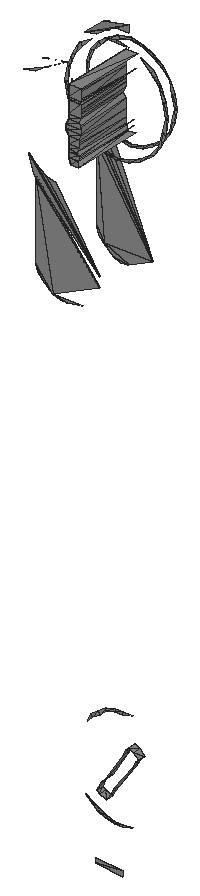
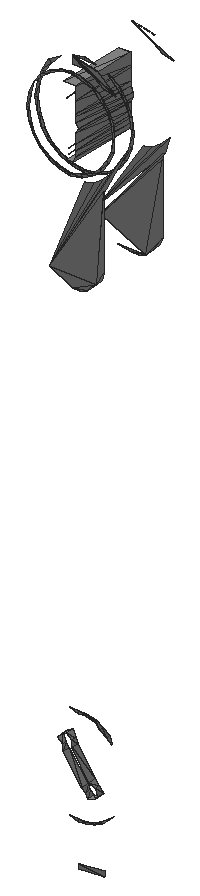
# SketchUp Ruby script. Lengths in inches.
U = 1.inch
M = Sketchup.active_model
def pt(a) = Geom::Point3d.new(a.map { |v| v * U })
def face(e, loops, mat)
  f = e.add_face(loops[0].map { |a| pt(a) })
  loops[1..].each { |l| e.add_face(l.map { |a| pt(a) }).erase! }
  f.material = f.back_material = mat if mat
  f
end
# faces: each face lists its corners as indices into pts; further lists are holes
def faces(e, pts, list, mat = nil) = list.each { |f| face(e, (f[0].is_a?(Array) ? f : [f]).map { |l| l.map { |i| pts[i] } }, mat) }
# xy, xz, yz: faces in a plane at the given z, y or x. An outline is a flat list of corners, or four numbers for a rectangle; further outlines are holes
def ring(l) = l.size == 4 ? [[l[0], l[1]], [l[2], l[1]], [l[2], l[3]], [l[0], l[3]]] : l.each_slice(2).to_a
def flat(e, list, mat, &to3) = list.each { |f| face(e, (f[0].is_a?(Array) ? f : [f]).map { |l| ring(l).map { |u, v| to3.(u, v) } }, mat) }
def xy(e, z, list, mat = nil) = flat(e, list, mat) { |x, y| [x, y, z] }
def xz(e, y, list, mat = nil) = flat(e, list, mat) { |x, z| [x, y, z] }
def yz(e, x, list, mat = nil) = flat(e, list, mat) { |y, z| [x, y, z] }
def lines(e, pts, list) = list.each { |a, b| e.add_line(pt(pts[a]), pt(pts[b])) }
# prism: a flat outline (further loops are holes) pulled along v
def prism(e, loops, v, mat = nil)
  f = face(e, loops, mat); d = Geom::Vector3d.new(v.map { |x| x * U })
  f.pushpull(f.normal.samedirection?(d) ? d.length : -d.length)
end
def box(e, o, s, mat = nil) = prism(e, [[o, [o[0] + s[0], o[1], o[2]], [o[0] + s[0], o[1] + s[1], o[2]], [o[0], o[1] + s[1], o[2]]]], [0, 0, s[2]], mat)
def at(x, y, z, deg = 0) = Geom::Transformation.translation(pt([x, y, z])) * Geom::Transformation.rotation(ORIGIN, Z_AXIS, deg.degrees)
def axes(o, x, y, z) = Geom::Transformation.new([*x, 0, *y, 0, *z, 0, *pt(o).to_a, 1])
def part(name) = M.definitions.add(name)
# library, detail: a bought-in or finely detailed component or shape, given as its bounding box
def library(name, o, s) = part(name).tap { |d| box(d.entities, o, s) }
def detail(e, o, s) = box(e.add_group.entities, o, s)
def put(e, d, t, mat = nil) = e.add_instance(d, t).tap { |i| i.material = mat if mat }
def group(e, t, mat = nil) = e.add_group.tap { |g| g.transformation = t; g.material = mat if mat }.entities
root = M.entities
M.materials.add("Material \#1").color = [140, 140, 140]
xy(root,161.124,[[359.541,200.864,359.541,201.153,359.571,200.864],[359.571,200.864,359.541,201.153,359.571,201.153]],"Material \#1")
xy(root,161.418,[[359.526,200.864,359.576,200.864,359.576,201.153],[359.526,200.864,359.576,201.153,359.526,201.153]],"Material \#1")
xz(root,200.833,[[359.551,160.635,359.494,160.65,359.609,160.65],[359.551,160.635,359.521,160.639,359.494,160.65],[359.494,160.65,359.42,161.042,359.679,160.743],[359.494,160.65,359.423,160.743,359.42,161.042],[359.494,160.65,359.449,160.688,359.423,160.743],
  [359.494,160.65,359.469,160.666,359.449,160.688],[359.449,160.688,359.433,160.714,359.423,160.743],[359.679,160.743,359.417,161.058,359.415,161.063],[359.679,160.743,359.419,161.053,359.417,161.058],[359.679,160.743,359.42,161.048,359.419,161.053],
  [359.423,160.743,359.42,160.775,359.42,161.042],[359.679,160.743,359.42,161.042,359.42,161.048],[359.682,160.775,359.39,161.133,359.422,161.099],[359.682,160.775,359.415,161.063,359.39,161.133],[359.682,160.775,359.422,161.099,359.46,161.073],
  [359.682,160.775,359.46,161.073,359.504,161.056],[359.368,161.427,359.46,161.469,359.422,161.443],[359.46,161.469,359.551,161.521,359.504,161.486],[359.448,161.495,359.497,161.514,359.551,161.521]],"Material \#1")
xz(root,200.864,[[359.541,161.124,359.561,161.146,359.531,161.146],[359.541,161.124,359.571,161.124,359.561,161.146],[359.531,161.146,359.567,161.153,359.526,161.153],[359.531,161.146,359.561,161.146,359.567,161.153],[359.526,161.153,359.567,161.153,359.567,161.17],
  [359.526,161.153,359.567,161.17,359.526,161.17],[359.526,161.17,359.561,161.177,359.531,161.177],[359.526,161.17,359.567,161.17,359.561,161.177],[359.531,161.177,359.561,161.177,359.571,161.205],[359.531,161.177,359.571,161.205,359.531,161.205],
  [359.531,161.205,359.571,161.205,359.571,161.231],[359.531,161.205,359.571,161.231,359.531,161.231],[359.531,161.231,359.579,161.251,359.524,161.251],[359.531,161.231,359.571,161.231,359.579,161.251],[359.524,161.251,359.579,161.251,359.579,161.272],
  [359.524,161.251,359.579,161.272,359.524,161.272],[359.524,161.272,359.571,161.293,359.531,161.293],[359.524,161.272,359.579,161.272,359.571,161.293],[359.531,161.293,359.576,161.308,359.526,161.308],[359.531,161.293,359.571,161.293,359.576,161.308],
  [359.526,161.308,359.576,161.308,359.576,161.356],[359.526,161.308,359.576,161.356,359.526,161.356],[359.526,161.356,359.57,161.359,359.533,161.359],[359.526,161.356,359.576,161.356,359.57,161.359],[359.533,161.359,359.57,161.359,359.57,161.367],
  [359.533,161.359,359.57,161.367,359.533,161.367],[359.533,161.367,359.576,161.37,359.526,161.37],[359.533,161.367,359.57,161.367,359.576,161.37],[359.526,161.37,359.576,161.37,359.576,161.418],[359.526,161.37,359.576,161.418,359.526,161.418]],"Material \#1")
xz(root,201.082,[[359.551,161.051,359.551,161.058,359.498,161.058],[359.551,161.051,359.603,161.065,359.551,161.058],[359.551,161.051,359.605,161.058,359.603,161.065],[359.498,161.058,359.499,161.065,359.448,161.08],[359.498,161.058,359.551,161.058,359.499,161.065],
  [359.605,161.058,359.651,161.087,359.603,161.065],[359.605,161.058,359.655,161.08,359.651,161.087],[359.499,161.065,359.451,161.087,359.448,161.08],[359.448,161.08,359.451,161.087,359.405,161.115],[359.655,161.08,359.693,161.12,359.651,161.087],
  [359.655,161.08,359.698,161.115,359.693,161.12],[359.451,161.087,359.41,161.12,359.405,161.115],[359.405,161.115,359.41,161.12,359.372,161.161],[359.698,161.115,359.725,161.165,359.693,161.12],[359.698,161.115,359.731,161.161,359.725,161.165],
  [359.41,161.12,359.378,161.165,359.372,161.161],[359.372,161.161,359.378,161.165,359.351,161.214],[359.731,161.161,359.745,161.216,359.725,161.165],[359.731,161.161,359.751,161.214,359.745,161.216],[359.378,161.165,359.358,161.216,359.351,161.214],
  [359.351,161.214,359.358,161.216,359.344,161.271],[359.751,161.214,359.751,161.271,359.745,161.216],[359.751,161.214,359.758,161.271,359.751,161.271],[359.358,161.216,359.351,161.271,359.344,161.271],[359.344,161.271,359.351,161.271,359.351,161.328],
  [359.351,161.271,359.358,161.326,359.351,161.328],[359.751,161.271,359.758,161.271,359.745,161.326],[359.758,161.271,359.751,161.328,359.745,161.326],[359.358,161.326,359.372,161.381,359.351,161.328],[359.358,161.326,359.378,161.378,359.372,161.381],
  [359.745,161.326,359.751,161.328,359.725,161.378],[359.751,161.328,359.731,161.381,359.725,161.378],[359.378,161.378,359.405,161.427,359.372,161.381],[359.378,161.378,359.41,161.422,359.405,161.427],[359.725,161.378,359.731,161.381,359.693,161.422],
  [359.731,161.381,359.698,161.427,359.693,161.422],[359.41,161.422,359.448,161.462,359.405,161.427],[359.41,161.422,359.451,161.456,359.448,161.462],[359.693,161.422,359.698,161.427,359.651,161.456],[359.698,161.427,359.655,161.462,359.651,161.456],
  [359.451,161.456,359.498,161.484,359.448,161.462],[359.451,161.456,359.499,161.477,359.498,161.484],[359.651,161.456,359.655,161.462,359.603,161.477],[359.655,161.462,359.605,161.484,359.603,161.477],[359.499,161.477,359.551,161.491,359.498,161.484],
  [359.499,161.477,359.551,161.484,359.551,161.491],[359.603,161.477,359.605,161.484,359.551,161.484],[359.551,161.484,359.605,161.484,359.551,161.491]],"Material \#1")
xz(root,201.113,[[359.551,158.424,359.551,158.435,359.443,158.434],[359.443,158.434,359.551,158.435,359.444,158.445],[359.551,158.596,359.551,158.607,359.515,158.599],[359.551,158.596,359.585,158.61,359.551,158.607],[359.515,158.599,359.517,158.61,359.481,158.609],
  [359.515,158.599,359.551,158.607,359.517,158.61],[359.481,158.609,359.485,158.62,359.45,158.625],[359.481,158.609,359.517,158.61,359.485,158.62],[359.485,158.62,359.455,158.635,359.45,158.625],[359.45,158.625,359.455,158.635,359.422,158.646],
  [359.455,158.635,359.429,158.655,359.422,158.646],[359.422,158.646,359.429,158.655,359.398,158.672],[359.406,158.94,359.429,158.964,359.422,158.973],[359.429,158.964,359.45,158.994,359.422,158.973],[359.429,158.964,359.455,158.984,359.45,158.994],
  [359.455,158.984,359.481,159.01,359.45,158.994],[359.455,158.984,359.485,158.999,359.481,159.01],[359.485,158.999,359.515,159.019,359.481,159.01],[359.485,158.999,359.517,159.009,359.515,159.019],[359.517,159.009,359.551,159.023,359.515,159.019],
  [359.517,159.009,359.551,159.012,359.551,159.023],[359.551,159.012,359.587,159.019,359.551,159.023]],"Material \#1")
xz(root,201.144,[[359.551,160.635,359.449,160.688,359.494,160.65],[359.551,160.635,359.654,160.688,359.449,160.688],[359.551,160.635,359.494,160.65,359.521,160.639],[359.494,160.65,359.449,160.688,359.469,160.666],[359.654,160.688,359.318,161.238,359.415,161.063],
  [359.654,160.688,359.39,161.133,359.318,161.238],[359.654,160.688,359.422,161.099,359.39,161.133],[359.654,160.688,359.415,161.063,359.417,161.058],[359.654,160.688,359.417,161.058,359.419,161.053],[359.654,160.688,359.419,161.053,359.42,161.048],
  [359.449,160.688,359.42,161.042,359.423,160.743],[359.449,160.688,359.42,161.048,359.42,161.042],[359.449,160.688,359.654,160.688,359.42,161.048],[359.654,160.688,359.46,161.073,359.422,161.099],[359.449,160.688,359.423,160.743,359.433,160.714],
  [359.654,160.688,359.504,161.056,359.46,161.073],[359.423,160.743,359.42,161.042,359.42,160.775],[359.368,161.427,359.422,161.443,359.46,161.469],[359.368,161.427,359.46,161.469,359.551,161.521],[359.368,161.427,359.551,161.521,359.448,161.495],
  [359.46,161.469,359.504,161.486,359.551,161.521],[359.504,161.486,359.551,161.491,359.551,161.521],[359.448,161.495,359.551,161.521,359.497,161.514]],"Material \#1")
xz(root,201.153,[[359.551,161.075,359.551,161.082,359.503,161.081],[359.551,161.075,359.597,161.088,359.551,161.082],[359.551,161.075,359.599,161.081,359.597,161.088],[359.503,161.081,359.505,161.088,359.459,161.101],[359.503,161.081,359.551,161.082,359.505,161.088],
  [359.599,161.081,359.64,161.107,359.597,161.088],[359.599,161.081,359.644,161.101,359.64,161.107],[359.505,161.088,359.462,161.107,359.459,161.101],[359.459,161.101,359.462,161.107,359.421,161.132],[359.644,161.101,359.677,161.137,359.64,161.107],
  [359.644,161.101,359.682,161.132,359.677,161.137],[359.462,161.107,359.426,161.137,359.421,161.132],[359.421,161.132,359.426,161.137,359.391,161.173],[359.682,161.132,359.705,161.176,359.677,161.137],[359.682,161.132,359.711,161.173,359.705,161.176],
  [359.426,161.137,359.397,161.176,359.391,161.173],[359.391,161.173,359.397,161.176,359.373,161.22],[359.711,161.173,359.723,161.222,359.705,161.176],[359.711,161.173,359.73,161.22,359.723,161.222],[359.397,161.176,359.38,161.222,359.373,161.22],
  [359.373,161.22,359.38,161.222,359.367,161.271],[359.73,161.22,359.729,161.271,359.723,161.222],[359.73,161.22,359.736,161.271,359.729,161.271],[359.38,161.222,359.374,161.271,359.367,161.271],[359.367,161.271,359.374,161.271,359.373,161.322],
  [359.374,161.271,359.38,161.32,359.373,161.322],[359.729,161.271,359.736,161.271,359.723,161.32],[359.736,161.271,359.73,161.322,359.723,161.32],[359.38,161.32,359.391,161.369,359.373,161.322],[359.38,161.32,359.397,161.366,359.391,161.369],
  [359.723,161.32,359.73,161.322,359.705,161.366],[359.73,161.322,359.711,161.369,359.705,161.366],[359.397,161.366,359.421,161.41,359.391,161.369],[359.397,161.366,359.426,161.405,359.421,161.41],[359.705,161.366,359.711,161.369,359.677,161.405],
  [359.711,161.369,359.682,161.41,359.677,161.405],[359.426,161.405,359.459,161.441,359.421,161.41],[359.426,161.405,359.462,161.435,359.459,161.441],[359.677,161.405,359.682,161.41,359.64,161.435],[359.682,161.41,359.644,161.441,359.64,161.435],
  [359.462,161.435,359.503,161.461,359.459,161.441],[359.462,161.435,359.505,161.454,359.503,161.461],[359.64,161.435,359.644,161.441,359.597,161.454],[359.644,161.441,359.599,161.461,359.597,161.454],[359.505,161.454,359.551,161.467,359.503,161.461],
  [359.505,161.454,359.551,161.46,359.551,161.467],[359.597,161.454,359.599,161.461,359.551,161.46],[359.551,161.46,359.599,161.461,359.551,161.467]],"Material \#1")
yz(root,359.526,[[200.864,161.37,200.864,161.418,201.153,161.418]],"Material \#1")
yz(root,359.531,[[200.864,161.177,200.864,161.205,201.153,161.205]],"Material \#1")
p = [[359.496,201.116,158.768],[359.482,201.113,158.748],[359.482,201.088,158.748],[359.496,201.091,158.768],[359.467,201.106,158.725],[359.467,201.081,158.725],
  [359.484,201.106,158.708],[359.484,201.081,158.708],[359.505,201.106,158.696],[359.505,201.081,158.696],[359.52,201.113,158.719],[359.52,201.088,158.719],
  [359.534,201.116,158.74],[359.534,201.091,158.74],[359.607,201.116,158.851],[359.607,201.091,158.851],[359.569,201.116,158.879],[359.569,201.091,158.879],
  [359.621,201.113,158.871],[359.621,201.088,158.871],[359.636,201.106,158.894],[359.636,201.081,158.894],[359.618,201.106,158.911],[359.618,201.081,158.911],
  [359.597,201.106,158.923],[359.597,201.081,158.923],[359.582,201.113,158.9],[359.582,201.088,158.9],[359.529,201.153,161.15],[359.541,201.153,161.124],
  [359.541,200.864,161.124],[359.531,200.864,161.146],[359.529,201.153,161.15],[359.529,201.153,161.15],[359.531,200.864,161.146],[359.526,200.864,161.153],
  [359.529,201.153,161.174],[359.529,201.153,161.15],[359.526,200.864,161.153],[359.564,201.153,161.15],[359.567,200.864,161.153],[359.561,200.864,161.146],
  [359.529,201.153,161.174],[359.526,200.864,161.17],[359.531,200.864,161.177],[359.531,200.864,161.231],[359.524,200.864,161.251],[359.524,201.153,161.262],
  [359.531,200.864,161.205],[359.531,200.864,161.231],[359.528,201.153,161.241],[359.526,200.864,161.17],[359.531,201.153,161.205],[359.529,201.153,161.174],
  [359.531,200.864,161.177],[359.524,201.153,161.262],[359.528,201.153,161.241],[359.531,200.864,161.231],[359.528,201.153,161.241],[359.531,201.153,161.205],
  [359.531,200.864,161.205],[359.564,201.153,161.174],[359.561,200.864,161.177],[359.567,200.864,161.17],[359.526,200.864,161.308],[359.526,200.864,161.356],
  [359.529,201.153,161.36],[359.531,200.864,161.293],[359.526,200.864,161.308],[359.527,201.153,161.311],[359.524,200.864,161.272],[359.531,200.864,161.293],
  [359.529,201.153,161.3],[359.524,200.864,161.251],[359.524,200.864,161.272],[359.528,201.153,161.283],[359.529,201.153,161.36],[359.527,201.153,161.311],
  [359.526,200.864,161.308],[359.527,201.153,161.311],[359.529,201.153,161.3],[359.531,200.864,161.293],[359.529,201.153,161.3],[359.528,201.153,161.283],
  [359.524,200.864,161.272],[359.528,201.153,161.283],[359.524,201.153,161.262],[359.524,200.864,161.251],[359.529,201.153,161.36],[359.533,200.864,161.359],
  [359.533,200.864,161.367],[359.529,201.153,161.36],[359.526,200.864,161.37],[359.529,201.153,161.36],[359.526,200.864,161.356],[359.526,201.153,161.418],
  [359.529,201.153,161.36],[359.526,200.864,161.37],[359.574,201.153,161.364],[359.57,200.864,161.359],[359.576,200.864,161.356],[359.574,201.153,161.364],
  [359.576,200.864,161.37],[359.57,200.864,161.367],[359.574,201.153,161.364]]
faces(root,p,[[0,1,2],[2,3,0],[1,4,5],[5,2,1],[4,6,7],[7,5,4],[6,8,9],[9,7,6],
  [8,10,11],[11,9,8],[10,12,13],[13,11,10],[12,14,15],[15,13,12],[16,0,3],[3,17,16],
  [14,18,19],[19,15,14],[18,20,21],[21,19,18],[20,22,23],[23,21,20],[22,24,25],[25,23,22],
  [24,26,27],[27,25,24],[26,16,17],[17,27,26],[28,29,30],[30,31,32],[33,34,35],[36,37,38],
  [39,40,41],[42,43,44],[45,46,47],[48,49,50],[38,51,36],[52,53,54],[55,56,57],[58,59,60],
  [61,62,63],[64,65,66],[67,68,69],[70,71,72],[73,74,75],[76,77,78],[79,80,81],[82,83,84],
  [85,86,87],[88,89,90],[91,90,92],[93,94,89],[95,96,97],[98,99,100],[101,102,103],[104,103,99]],"Material \#1")
